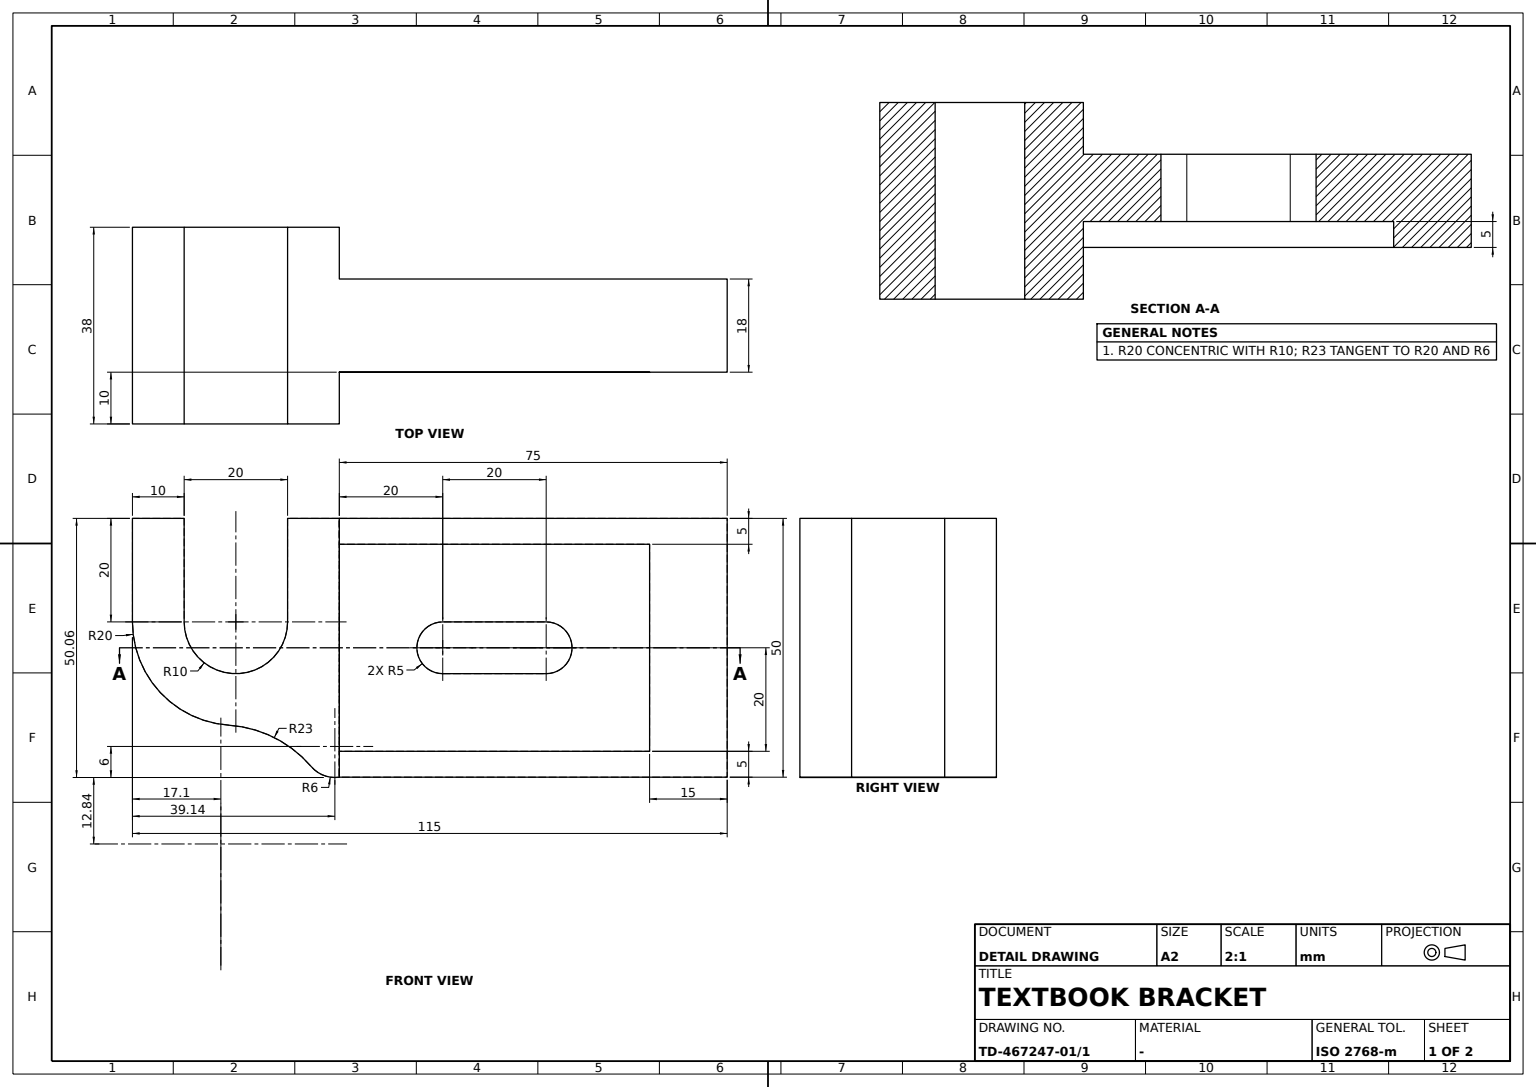
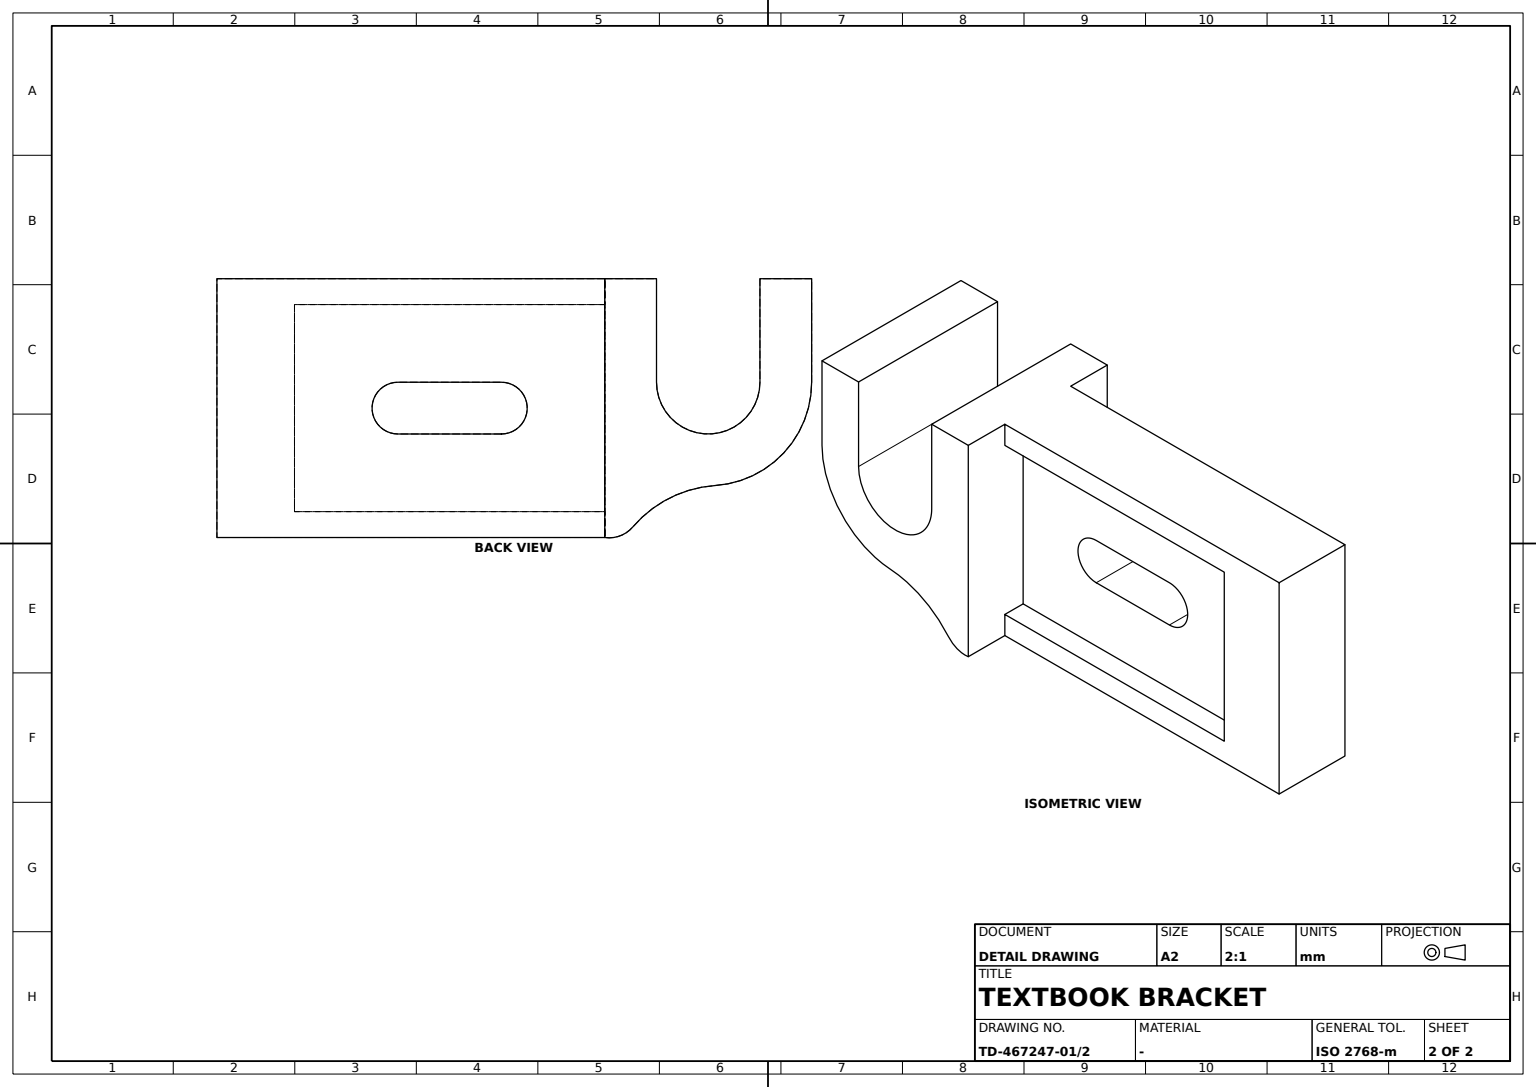
ISO-10303-21;
HEADER;
FILE_DESCRIPTION((''),'2;1');
FILE_NAME('','',(''),(''),'','','');
FILE_SCHEMA(('AUTOMOTIVE_DESIGN'));
ENDSEC;
DATA;
#1=APPLICATION_CONTEXT('');
#2=PRODUCT_CONTEXT('',#1,'mechanical');
#3=PRODUCT('','','',(#2));
#4=PRODUCT_DEFINITION_FORMATION('','',#3);
#5=PRODUCT_DEFINITION_CONTEXT('',#1,'design');
#6=PRODUCT_DEFINITION('','',#4,#5);
#7=PRODUCT_DEFINITION_SHAPE('','',#6);
#8=(LENGTH_UNIT()NAMED_UNIT(*)SI_UNIT(.MILLI.,.METRE.));
#9=(NAMED_UNIT(*)PLANE_ANGLE_UNIT()SI_UNIT($,.RADIAN.));
#10=(NAMED_UNIT(*)SI_UNIT($,.STERADIAN.)SOLID_ANGLE_UNIT());
#11=UNCERTAINTY_MEASURE_WITH_UNIT(LENGTH_MEASURE(0.005),#8,'distance_accuracy_value','');
#12=(GEOMETRIC_REPRESENTATION_CONTEXT(3)GLOBAL_UNCERTAINTY_ASSIGNED_CONTEXT((#11))GLOBAL_UNIT_ASSIGNED_CONTEXT((#8,#9,#10))REPRESENTATION_CONTEXT('',''));
#13=CARTESIAN_POINT('',(19.,-5.417023,-22.959402));
#14=VERTEX_POINT('',#13);
#15=CARTESIAN_POINT('',(19.,0.,-25.));
#16=VERTEX_POINT('',#15);
#17=CARTESIAN_POINT('',(19.,-0.85576,-19.061341));
#18=DIRECTION('',(1.,0.,0.));
#19=DIRECTION('',(0.,0.,-1.));
#20=AXIS2_PLACEMENT_3D('',#17,#18,#19);
#21=CIRCLE('',#20,6.);
#22=EDGE_CURVE('',#14,#16,#21,.T.);
#23=ORIENTED_EDGE('',*,*,#22,.F.);
#24=CARTESIAN_POINT('',(-19.,-5.417023,-22.959402));
#25=VERTEX_POINT('',#24);
#26=CARTESIAN_POINT('',(0.,-5.417023,-22.959402));
#27=VECTOR('',#18,1000.);
#28=LINE('',#26,#27);
#29=EDGE_CURVE('',#25,#14,#28,.T.);
#30=ORIENTED_EDGE('',*,*,#29,.F.);
#31=CARTESIAN_POINT('',(-19.,0.,-25.));
#32=VERTEX_POINT('',#31);
#33=CARTESIAN_POINT('',(-19.,-0.85576,-19.061341));
#34=AXIS2_PLACEMENT_3D('',#33,#18,#19);
#35=CIRCLE('',#34,6.);
#36=EDGE_CURVE('',#25,#32,#35,.T.);
#37=ORIENTED_EDGE('',*,*,#36,.T.);
#38=CARTESIAN_POINT('',(-9.,0.,-25.));
#39=VERTEX_POINT('',#38);
#40=LINE('',#31,#27);
#41=EDGE_CURVE('',#32,#39,#40,.T.);
#42=ORIENTED_EDGE('',*,*,#41,.T.);
#43=CARTESIAN_POINT('',(9.,0.,-25.));
#44=VERTEX_POINT('',#43);
#45=LINE('',#38,#27);
#46=EDGE_CURVE('',#39,#44,#45,.T.);
#47=ORIENTED_EDGE('',*,*,#46,.T.);
#48=LINE('',#43,#27);
#49=EDGE_CURVE('',#44,#16,#48,.T.);
#50=ORIENTED_EDGE('',*,*,#49,.T.);
#51=EDGE_LOOP('',(#23,#30,#37,#42,#47,#50));
#52=FACE_BOUND('',#51,.T.);
#53=CARTESIAN_POINT('',(0.,-0.85576,-19.061341));
#54=DIRECTION('',(0.,1.,0.));
#55=AXIS2_PLACEMENT_3D('',#53,#18,#54);
#56=CYLINDRICAL_SURFACE('',#55,6.);
#57=ADVANCED_FACE('',(#52),#56,.T.);
#58=CARTESIAN_POINT('',(-19.,-21.349703,-14.954406));
#59=VERTEX_POINT('',#58);
#60=CARTESIAN_POINT('',(19.,-21.349703,-14.954406));
#61=VERTEX_POINT('',#60);
#62=CARTESIAN_POINT('',(0.,-21.349703,-14.954406));
#63=LINE('',#62,#27);
#64=EDGE_CURVE('',#59,#61,#63,.T.);
#65=ORIENTED_EDGE('',*,*,#64,.T.);
#66=CARTESIAN_POINT('',(19.,-40.,5.));
#67=VERTEX_POINT('',#66);
#68=CARTESIAN_POINT('',(19.,-20.,5.));
#69=AXIS2_PLACEMENT_3D('',#68,#18,#19);
#70=CIRCLE('',#69,20.);
#71=EDGE_CURVE('',#67,#61,#70,.T.);
#72=ORIENTED_EDGE('',*,*,#71,.F.);
#73=CARTESIAN_POINT('',(-19.,-40.,5.));
#74=VERTEX_POINT('',#73);
#75=CARTESIAN_POINT('',(0.,-40.,5.));
#76=LINE('',#75,#27);
#77=EDGE_CURVE('',#74,#67,#76,.T.);
#78=ORIENTED_EDGE('',*,*,#77,.F.);
#79=CARTESIAN_POINT('',(-19.,-20.,5.));
#80=AXIS2_PLACEMENT_3D('',#79,#18,#19);
#81=CIRCLE('',#80,20.);
#82=EDGE_CURVE('',#74,#59,#81,.T.);
#83=ORIENTED_EDGE('',*,*,#82,.T.);
#84=EDGE_LOOP('',(#65,#72,#78,#83));
#85=FACE_BOUND('',#84,.T.);
#86=CARTESIAN_POINT('',(0.,-20.,5.));
#87=AXIS2_PLACEMENT_3D('',#86,#18,#54);
#88=CYLINDRICAL_SURFACE('',#87,20.);
#89=ADVANCED_FACE('',(#85),#88,.T.);
#90=CARTESIAN_POINT('',(4.,0.,20.));
#91=VERTEX_POINT('',#90);
#92=CARTESIAN_POINT('',(4.,60.,20.));
#93=VERTEX_POINT('',#92);
#94=VECTOR('',#54,1000.);
#95=LINE('',#90,#94);
#96=EDGE_CURVE('',#91,#93,#95,.T.);
#97=ORIENTED_EDGE('',*,*,#96,.T.);
#98=CARTESIAN_POINT('',(9.,60.,20.));
#99=VERTEX_POINT('',#98);
#100=DIRECTION('',(-1.,0.,0.));
#101=VECTOR('',#100,1000.);
#102=LINE('',#98,#101);
#103=EDGE_CURVE('',#99,#93,#102,.T.);
#104=ORIENTED_EDGE('',*,*,#103,.F.);
#105=CARTESIAN_POINT('',(9.,0.,20.));
#106=VERTEX_POINT('',#105);
#107=LINE('',#105,#94);
#108=EDGE_CURVE('',#106,#99,#107,.T.);
#109=ORIENTED_EDGE('',*,*,#108,.F.);
#110=LINE('',#105,#27);
#111=EDGE_CURVE('',#91,#106,#110,.T.);
#112=ORIENTED_EDGE('',*,*,#111,.F.);
#113=EDGE_LOOP('',(#97,#104,#109,#112));
#114=FACE_BOUND('',#113,.T.);
#115=DIRECTION('',(0.,0.,1.));
#116=AXIS2_PLACEMENT_3D('',#105,#115,#54);
#117=PLANE('',#116);
#118=ADVANCED_FACE('',(#114),#117,.F.);
#119=CARTESIAN_POINT('',(-19.,-10.,5.));
#120=VERTEX_POINT('',#119);
#121=CARTESIAN_POINT('',(-19.,-10.,25.));
#122=VERTEX_POINT('',#121);
#123=CARTESIAN_POINT('',(-19.,-10.,0.));
#124=VECTOR('',#115,1000.);
#125=LINE('',#123,#124);
#126=EDGE_CURVE('',#120,#122,#125,.T.);
#127=ORIENTED_EDGE('',*,*,#126,.F.);
#128=CARTESIAN_POINT('',(19.,-10.,5.));
#129=VERTEX_POINT('',#128);
#130=CARTESIAN_POINT('',(0.,-10.,5.));
#131=LINE('',#130,#27);
#132=EDGE_CURVE('',#120,#129,#131,.T.);
#133=ORIENTED_EDGE('',*,*,#132,.T.);
#134=CARTESIAN_POINT('',(19.,-10.,25.));
#135=VERTEX_POINT('',#134);
#136=CARTESIAN_POINT('',(19.,-10.,0.));
#137=LINE('',#136,#124);
#138=EDGE_CURVE('',#129,#135,#137,.T.);
#139=ORIENTED_EDGE('',*,*,#138,.T.);
#140=CARTESIAN_POINT('',(0.,-10.,25.));
#141=LINE('',#140,#27);
#142=EDGE_CURVE('',#122,#135,#141,.T.);
#143=ORIENTED_EDGE('',*,*,#142,.F.);
#144=EDGE_LOOP('',(#127,#133,#139,#143));
#145=FACE_BOUND('',#144,.T.);
#146=AXIS2_PLACEMENT_3D('',#130,#54,#115);
#147=PLANE('',#146);
#148=ADVANCED_FACE('',(#145),#147,.F.);
#149=CARTESIAN_POINT('',(9.,60.,-20.));
#150=VERTEX_POINT('',#149);
#151=VECTOR('',#19,1000.);
#152=LINE('',#98,#151);
#153=EDGE_CURVE('',#99,#150,#152,.T.);
#154=ORIENTED_EDGE('',*,*,#153,.F.);
#155=ORIENTED_EDGE('',*,*,#103,.T.);
#156=CARTESIAN_POINT('',(4.,60.,-20.));
#157=VERTEX_POINT('',#156);
#158=LINE('',#92,#151);
#159=EDGE_CURVE('',#93,#157,#158,.T.);
#160=ORIENTED_EDGE('',*,*,#159,.T.);
#161=LINE('',#149,#101);
#162=EDGE_CURVE('',#150,#157,#161,.T.);
#163=ORIENTED_EDGE('',*,*,#162,.F.);
#164=EDGE_LOOP('',(#154,#155,#160,#163));
#165=FACE_BOUND('',#164,.T.);
#166=AXIS2_PLACEMENT_3D('',#98,#54,#19);
#167=PLANE('',#166);
#168=ADVANCED_FACE('',(#165),#167,.F.);
#169=CARTESIAN_POINT('',(-9.,0.,25.));
#170=VERTEX_POINT('',#169);
#171=CARTESIAN_POINT('',(-9.,0.,0.));
#172=LINE('',#171,#151);
#173=EDGE_CURVE('',#170,#39,#172,.T.);
#174=ORIENTED_EDGE('',*,*,#173,.F.);
#175=CARTESIAN_POINT('',(-9.,75.,25.));
#176=VERTEX_POINT('',#175);
#177=LINE('',#169,#94);
#178=EDGE_CURVE('',#170,#176,#177,.T.);
#179=ORIENTED_EDGE('',*,*,#178,.T.);
#180=CARTESIAN_POINT('',(-9.,75.,-25.));
#181=VERTEX_POINT('',#180);
#182=CARTESIAN_POINT('',(-9.,75.,0.));
#183=LINE('',#182,#124);
#184=EDGE_CURVE('',#181,#176,#183,.T.);
#185=ORIENTED_EDGE('',*,*,#184,.F.);
#186=DIRECTION('',(0.,-1.,0.));
#187=VECTOR('',#186,1000.);
#188=LINE('',#38,#187);
#189=EDGE_CURVE('',#181,#39,#188,.T.);
#190=ORIENTED_EDGE('',*,*,#189,.T.);
#191=EDGE_LOOP('',(#174,#179,#185,#190));
#192=FACE_BOUND('',#191,.T.);
#193=CARTESIAN_POINT('',(-9.,20.,5.));
#194=VERTEX_POINT('',#193);
#195=CARTESIAN_POINT('',(-9.,40.,5.));
#196=VERTEX_POINT('',#195);
#197=LINE('',#193,#94);
#198=EDGE_CURVE('',#194,#196,#197,.T.);
#199=ORIENTED_EDGE('',*,*,#198,.F.);
#200=CARTESIAN_POINT('',(-9.,20.,-5.));
#201=VERTEX_POINT('',#200);
#202=CARTESIAN_POINT('',(-9.,20.,0.));
#203=AXIS2_PLACEMENT_3D('',#202,#18,#19);
#204=CIRCLE('',#203,5.);
#205=EDGE_CURVE('',#194,#201,#204,.T.);
#206=ORIENTED_EDGE('',*,*,#205,.T.);
#207=CARTESIAN_POINT('',(-9.,40.,-5.));
#208=VERTEX_POINT('',#207);
#209=LINE('',#200,#94);
#210=EDGE_CURVE('',#201,#208,#209,.T.);
#211=ORIENTED_EDGE('',*,*,#210,.T.);
#212=CARTESIAN_POINT('',(-9.,40.,0.));
#213=AXIS2_PLACEMENT_3D('',#212,#18,#19);
#214=CIRCLE('',#213,5.);
#215=EDGE_CURVE('',#208,#196,#214,.T.);
#216=ORIENTED_EDGE('',*,*,#215,.T.);
#217=EDGE_LOOP('',(#199,#206,#211,#216));
#218=FACE_BOUND('',#217,.T.);
#219=AXIS2_PLACEMENT_3D('',#171,#18,#54);
#220=PLANE('',#219);
#221=ADVANCED_FACE('',(#192,#218),#220,.F.);
#222=CARTESIAN_POINT('',(4.,40.,-5.));
#223=VERTEX_POINT('',#222);
#224=CARTESIAN_POINT('',(-3.16,40.,-5.));
#225=LINE('',#224,#27);
#226=EDGE_CURVE('',#223,#208,#225,.F.);
#227=ORIENTED_EDGE('',*,*,#226,.F.);
#228=CARTESIAN_POINT('',(4.,40.,5.));
#229=VERTEX_POINT('',#228);
#230=CARTESIAN_POINT('',(4.,40.,0.));
#231=AXIS2_PLACEMENT_3D('',#230,#18,#19);
#232=CIRCLE('',#231,5.);
#233=EDGE_CURVE('',#223,#229,#232,.T.);
#234=ORIENTED_EDGE('',*,*,#233,.T.);
#235=CARTESIAN_POINT('',(-3.16,40.,5.));
#236=LINE('',#235,#27);
#237=EDGE_CURVE('',#229,#196,#236,.F.);
#238=ORIENTED_EDGE('',*,*,#237,.T.);
#239=ORIENTED_EDGE('',*,*,#215,.F.);
#240=EDGE_LOOP('',(#227,#234,#238,#239));
#241=FACE_BOUND('',#240,.T.);
#242=CARTESIAN_POINT('',(-3.16,40.,0.));
#243=AXIS2_PLACEMENT_3D('',#242,#18,#54);
#244=CYLINDRICAL_SURFACE('',#243,5.);
#245=ADVANCED_FACE('',(#241),#244,.F.);
#246=CARTESIAN_POINT('',(9.,75.,25.));
#247=VERTEX_POINT('',#246);
#248=CARTESIAN_POINT('',(0.,75.,25.));
#249=LINE('',#248,#27);
#250=EDGE_CURVE('',#176,#247,#249,.T.);
#251=ORIENTED_EDGE('',*,*,#250,.T.);
#252=CARTESIAN_POINT('',(9.,75.,-25.));
#253=VERTEX_POINT('',#252);
#254=CARTESIAN_POINT('',(9.,75.,0.));
#255=LINE('',#254,#124);
#256=EDGE_CURVE('',#253,#247,#255,.T.);
#257=ORIENTED_EDGE('',*,*,#256,.F.);
#258=CARTESIAN_POINT('',(0.,75.,-25.));
#259=LINE('',#258,#27);
#260=EDGE_CURVE('',#181,#253,#259,.T.);
#261=ORIENTED_EDGE('',*,*,#260,.F.);
#262=ORIENTED_EDGE('',*,*,#184,.T.);
#263=EDGE_LOOP('',(#251,#257,#261,#262));
#264=FACE_BOUND('',#263,.T.);
#265=AXIS2_PLACEMENT_3D('',#258,#54,#115);
#266=PLANE('',#265);
#267=ADVANCED_FACE('',(#264),#266,.T.);
#268=CARTESIAN_POINT('',(-19.,-40.,25.));
#269=VERTEX_POINT('',#268);
#270=CARTESIAN_POINT('',(19.,-40.,25.));
#271=VERTEX_POINT('',#270);
#272=CARTESIAN_POINT('',(0.,-40.,25.));
#273=LINE('',#272,#27);
#274=EDGE_CURVE('',#269,#271,#273,.T.);
#275=ORIENTED_EDGE('',*,*,#274,.F.);
#276=CARTESIAN_POINT('',(-19.,-40.,0.));
#277=LINE('',#276,#124);
#278=EDGE_CURVE('',#74,#269,#277,.T.);
#279=ORIENTED_EDGE('',*,*,#278,.F.);
#280=ORIENTED_EDGE('',*,*,#77,.T.);
#281=CARTESIAN_POINT('',(19.,-40.,0.));
#282=LINE('',#281,#124);
#283=EDGE_CURVE('',#67,#271,#282,.T.);
#284=ORIENTED_EDGE('',*,*,#283,.T.);
#285=EDGE_LOOP('',(#275,#279,#280,#284));
#286=FACE_BOUND('',#285,.T.);
#287=AXIS2_PLACEMENT_3D('',#75,#54,#115);
#288=PLANE('',#287);
#289=ADVANCED_FACE('',(#286),#288,.F.);
#290=ORIENTED_EDGE('',*,*,#198,.T.);
#291=ORIENTED_EDGE('',*,*,#237,.F.);
#292=CARTESIAN_POINT('',(4.,20.,5.));
#293=VERTEX_POINT('',#292);
#294=LINE('',#292,#94);
#295=EDGE_CURVE('',#293,#229,#294,.T.);
#296=ORIENTED_EDGE('',*,*,#295,.F.);
#297=CARTESIAN_POINT('',(-3.16,20.,5.));
#298=LINE('',#297,#27);
#299=EDGE_CURVE('',#293,#194,#298,.F.);
#300=ORIENTED_EDGE('',*,*,#299,.T.);
#301=EDGE_LOOP('',(#290,#291,#296,#300));
#302=FACE_BOUND('',#301,.T.);
#303=AXIS2_PLACEMENT_3D('',#292,#115,#54);
#304=PLANE('',#303);
#305=ADVANCED_FACE('',(#302),#304,.F.);
#306=CARTESIAN_POINT('',(-19.,-30.,5.));
#307=VERTEX_POINT('',#306);
#308=CIRCLE('',#80,10.);
#309=EDGE_CURVE('',#307,#120,#308,.T.);
#310=ORIENTED_EDGE('',*,*,#309,.F.);
#311=CARTESIAN_POINT('',(19.,-30.,5.));
#312=VERTEX_POINT('',#311);
#313=CARTESIAN_POINT('',(0.,-30.,5.));
#314=LINE('',#313,#27);
#315=EDGE_CURVE('',#307,#312,#314,.T.);
#316=ORIENTED_EDGE('',*,*,#315,.T.);
#317=CIRCLE('',#69,10.);
#318=EDGE_CURVE('',#312,#129,#317,.T.);
#319=ORIENTED_EDGE('',*,*,#318,.T.);
#320=ORIENTED_EDGE('',*,*,#132,.F.);
#321=EDGE_LOOP('',(#310,#316,#319,#320));
#322=FACE_BOUND('',#321,.T.);
#323=CYLINDRICAL_SURFACE('',#87,10.);
#324=ADVANCED_FACE('',(#322),#323,.F.);
#325=CARTESIAN_POINT('',(4.,20.,-5.));
#326=VERTEX_POINT('',#325);
#327=CARTESIAN_POINT('',(4.,20.,0.));
#328=AXIS2_PLACEMENT_3D('',#327,#18,#19);
#329=CIRCLE('',#328,5.);
#330=EDGE_CURVE('',#293,#326,#329,.T.);
#331=ORIENTED_EDGE('',*,*,#330,.T.);
#332=CARTESIAN_POINT('',(-3.16,20.,-5.));
#333=LINE('',#332,#27);
#334=EDGE_CURVE('',#326,#201,#333,.F.);
#335=ORIENTED_EDGE('',*,*,#334,.T.);
#336=ORIENTED_EDGE('',*,*,#205,.F.);
#337=ORIENTED_EDGE('',*,*,#299,.F.);
#338=EDGE_LOOP('',(#331,#335,#336,#337));
#339=FACE_BOUND('',#338,.T.);
#340=CARTESIAN_POINT('',(-3.16,20.,0.));
#341=AXIS2_PLACEMENT_3D('',#340,#18,#54);
#342=CYLINDRICAL_SURFACE('',#341,5.);
#343=ADVANCED_FACE('',(#339),#342,.F.);
#344=ORIENTED_EDGE('',*,*,#64,.F.);
#345=CARTESIAN_POINT('',(-19.,-22.901862,-37.901972));
#346=AXIS2_PLACEMENT_3D('',#345,#18,#19);
#347=CIRCLE('',#346,23.);
#348=EDGE_CURVE('',#25,#59,#347,.T.);
#349=ORIENTED_EDGE('',*,*,#348,.F.);
#350=ORIENTED_EDGE('',*,*,#29,.T.);
#351=CARTESIAN_POINT('',(19.,-22.901862,-37.901972));
#352=AXIS2_PLACEMENT_3D('',#351,#18,#19);
#353=CIRCLE('',#352,23.);
#354=EDGE_CURVE('',#14,#61,#353,.T.);
#355=ORIENTED_EDGE('',*,*,#354,.T.);
#356=EDGE_LOOP('',(#344,#349,#350,#355));
#357=FACE_BOUND('',#356,.T.);
#358=CARTESIAN_POINT('',(0.,-22.901862,-37.901972));
#359=AXIS2_PLACEMENT_3D('',#358,#18,#54);
#360=CYLINDRICAL_SURFACE('',#359,23.);
#361=ADVANCED_FACE('',(#357),#360,.F.);
#362=CARTESIAN_POINT('',(9.,0.,25.));
#363=VERTEX_POINT('',#362);
#364=CARTESIAN_POINT('',(19.,0.,25.));
#365=VERTEX_POINT('',#364);
#366=CARTESIAN_POINT('',(0.,0.,25.));
#367=LINE('',#366,#27);
#368=EDGE_CURVE('',#363,#365,#367,.T.);
#369=ORIENTED_EDGE('',*,*,#368,.F.);
#370=LINE('',#362,#94);
#371=EDGE_CURVE('',#363,#247,#370,.T.);
#372=ORIENTED_EDGE('',*,*,#371,.T.);
#373=ORIENTED_EDGE('',*,*,#250,.F.);
#374=ORIENTED_EDGE('',*,*,#178,.F.);
#375=CARTESIAN_POINT('',(-19.,0.,25.));
#376=VERTEX_POINT('',#375);
#377=EDGE_CURVE('',#376,#170,#367,.T.);
#378=ORIENTED_EDGE('',*,*,#377,.F.);
#379=LINE('',#375,#94);
#380=EDGE_CURVE('',#122,#376,#379,.T.);
#381=ORIENTED_EDGE('',*,*,#380,.F.);
#382=ORIENTED_EDGE('',*,*,#142,.T.);
#383=LINE('',#364,#94);
#384=EDGE_CURVE('',#135,#365,#383,.T.);
#385=ORIENTED_EDGE('',*,*,#384,.T.);
#386=EDGE_LOOP('',(#369,#372,#373,#374,#378,#381,#382,#385));
#387=FACE_BOUND('',#386,.T.);
#388=AXIS2_PLACEMENT_3D('',#366,#19,#54);
#389=PLANE('',#388);
#390=ADVANCED_FACE('',(#387),#389,.F.);
#391=CARTESIAN_POINT('',(19.,-30.,25.));
#392=VERTEX_POINT('',#391);
#393=CARTESIAN_POINT('',(19.,-30.,0.));
#394=LINE('',#393,#124);
#395=EDGE_CURVE('',#312,#392,#394,.T.);
#396=ORIENTED_EDGE('',*,*,#395,.F.);
#397=ORIENTED_EDGE('',*,*,#315,.F.);
#398=CARTESIAN_POINT('',(-19.,-30.,25.));
#399=VERTEX_POINT('',#398);
#400=CARTESIAN_POINT('',(-19.,-30.,0.));
#401=LINE('',#400,#124);
#402=EDGE_CURVE('',#307,#399,#401,.T.);
#403=ORIENTED_EDGE('',*,*,#402,.T.);
#404=CARTESIAN_POINT('',(0.,-30.,25.));
#405=LINE('',#404,#27);
#406=EDGE_CURVE('',#399,#392,#405,.T.);
#407=ORIENTED_EDGE('',*,*,#406,.T.);
#408=EDGE_LOOP('',(#396,#397,#403,#407));
#409=FACE_BOUND('',#408,.T.);
#410=AXIS2_PLACEMENT_3D('',#313,#54,#115);
#411=PLANE('',#410);
#412=ADVANCED_FACE('',(#409),#411,.T.);
#413=ORIENTED_EDGE('',*,*,#334,.F.);
#414=LINE('',#325,#94);
#415=EDGE_CURVE('',#326,#223,#414,.T.);
#416=ORIENTED_EDGE('',*,*,#415,.T.);
#417=ORIENTED_EDGE('',*,*,#226,.T.);
#418=ORIENTED_EDGE('',*,*,#210,.F.);
#419=EDGE_LOOP('',(#413,#416,#417,#418));
#420=FACE_BOUND('',#419,.T.);
#421=AXIS2_PLACEMENT_3D('',#325,#115,#54);
#422=PLANE('',#421);
#423=ADVANCED_FACE('',(#420),#422,.T.);
#424=ORIENTED_EDGE('',*,*,#415,.F.);
#425=ORIENTED_EDGE('',*,*,#330,.F.);
#426=ORIENTED_EDGE('',*,*,#295,.T.);
#427=ORIENTED_EDGE('',*,*,#233,.F.);
#428=EDGE_LOOP('',(#424,#425,#426,#427));
#429=FACE_BOUND('',#428,.T.);
#430=ORIENTED_EDGE('',*,*,#96,.F.);
#431=CARTESIAN_POINT('',(4.,0.,-20.));
#432=VERTEX_POINT('',#431);
#433=CARTESIAN_POINT('',(4.,0.,0.));
#434=LINE('',#433,#151);
#435=EDGE_CURVE('',#91,#432,#434,.T.);
#436=ORIENTED_EDGE('',*,*,#435,.T.);
#437=LINE('',#156,#187);
#438=EDGE_CURVE('',#157,#432,#437,.T.);
#439=ORIENTED_EDGE('',*,*,#438,.F.);
#440=ORIENTED_EDGE('',*,*,#159,.F.);
#441=EDGE_LOOP('',(#430,#436,#439,#440));
#442=FACE_BOUND('',#441,.T.);
#443=AXIS2_PLACEMENT_3D('',#433,#18,#54);
#444=PLANE('',#443);
#445=ADVANCED_FACE('',(#429,#442),#444,.T.);
#446=ORIENTED_EDGE('',*,*,#126,.T.);
#447=ORIENTED_EDGE('',*,*,#380,.T.);
#448=CARTESIAN_POINT('',(-19.,0.,0.));
#449=LINE('',#448,#151);
#450=EDGE_CURVE('',#376,#32,#449,.T.);
#451=ORIENTED_EDGE('',*,*,#450,.T.);
#452=ORIENTED_EDGE('',*,*,#36,.F.);
#453=ORIENTED_EDGE('',*,*,#348,.T.);
#454=ORIENTED_EDGE('',*,*,#82,.F.);
#455=ORIENTED_EDGE('',*,*,#278,.T.);
#456=EDGE_CURVE('',#269,#399,#379,.T.);
#457=ORIENTED_EDGE('',*,*,#456,.T.);
#458=ORIENTED_EDGE('',*,*,#402,.F.);
#459=ORIENTED_EDGE('',*,*,#309,.T.);
#460=EDGE_LOOP('',(#446,#447,#451,#452,#453,#454,#455,#457,#458,#459));
#461=FACE_BOUND('',#460,.T.);
#462=AXIS2_PLACEMENT_3D('',#448,#18,#54);
#463=PLANE('',#462);
#464=ADVANCED_FACE('',(#461),#463,.F.);
#465=CARTESIAN_POINT('',(9.,0.,-20.));
#466=VERTEX_POINT('',#465);
#467=LINE('',#149,#187);
#468=EDGE_CURVE('',#150,#466,#467,.T.);
#469=ORIENTED_EDGE('',*,*,#468,.F.);
#470=ORIENTED_EDGE('',*,*,#162,.T.);
#471=ORIENTED_EDGE('',*,*,#438,.T.);
#472=CARTESIAN_POINT('',(0.,0.,-20.));
#473=LINE('',#472,#27);
#474=EDGE_CURVE('',#432,#466,#473,.T.);
#475=ORIENTED_EDGE('',*,*,#474,.T.);
#476=EDGE_LOOP('',(#469,#470,#471,#475));
#477=FACE_BOUND('',#476,.T.);
#478=AXIS2_PLACEMENT_3D('',#149,#19,#186);
#479=PLANE('',#478);
#480=ADVANCED_FACE('',(#477),#479,.F.);
#481=ORIENTED_EDGE('',*,*,#173,.T.);
#482=ORIENTED_EDGE('',*,*,#41,.F.);
#483=ORIENTED_EDGE('',*,*,#450,.F.);
#484=ORIENTED_EDGE('',*,*,#377,.T.);
#485=EDGE_LOOP('',(#481,#482,#483,#484));
#486=FACE_BOUND('',#485,.T.);
#487=AXIS2_PLACEMENT_3D('',#366,#186,#19);
#488=PLANE('',#487);
#489=ADVANCED_FACE('',(#486),#488,.F.);
#490=ORIENTED_EDGE('',*,*,#189,.F.);
#491=ORIENTED_EDGE('',*,*,#260,.T.);
#492=LINE('',#43,#187);
#493=EDGE_CURVE('',#253,#44,#492,.T.);
#494=ORIENTED_EDGE('',*,*,#493,.T.);
#495=ORIENTED_EDGE('',*,*,#46,.F.);
#496=EDGE_LOOP('',(#490,#491,#494,#495));
#497=FACE_BOUND('',#496,.T.);
#498=AXIS2_PLACEMENT_3D('',#258,#115,#186);
#499=PLANE('',#498);
#500=ADVANCED_FACE('',(#497),#499,.F.);
#501=ORIENTED_EDGE('',*,*,#49,.F.);
#502=CARTESIAN_POINT('',(9.,0.,0.));
#503=LINE('',#502,#151);
#504=EDGE_CURVE('',#466,#44,#503,.T.);
#505=ORIENTED_EDGE('',*,*,#504,.F.);
#506=ORIENTED_EDGE('',*,*,#474,.F.);
#507=ORIENTED_EDGE('',*,*,#435,.F.);
#508=ORIENTED_EDGE('',*,*,#111,.T.);
#509=EDGE_CURVE('',#363,#106,#503,.T.);
#510=ORIENTED_EDGE('',*,*,#509,.F.);
#511=ORIENTED_EDGE('',*,*,#368,.T.);
#512=CARTESIAN_POINT('',(19.,0.,0.));
#513=LINE('',#512,#151);
#514=EDGE_CURVE('',#365,#16,#513,.T.);
#515=ORIENTED_EDGE('',*,*,#514,.T.);
#516=EDGE_LOOP('',(#501,#505,#506,#507,#508,#510,#511,#515));
#517=FACE_BOUND('',#516,.T.);
#518=ADVANCED_FACE('',(#517),#488,.F.);
#519=ORIENTED_EDGE('',*,*,#456,.F.);
#520=ORIENTED_EDGE('',*,*,#274,.T.);
#521=EDGE_CURVE('',#271,#392,#383,.T.);
#522=ORIENTED_EDGE('',*,*,#521,.T.);
#523=ORIENTED_EDGE('',*,*,#406,.F.);
#524=EDGE_LOOP('',(#519,#520,#522,#523));
#525=FACE_BOUND('',#524,.T.);
#526=ADVANCED_FACE('',(#525),#389,.F.);
#527=ORIENTED_EDGE('',*,*,#493,.F.);
#528=ORIENTED_EDGE('',*,*,#256,.T.);
#529=ORIENTED_EDGE('',*,*,#371,.F.);
#530=ORIENTED_EDGE('',*,*,#509,.T.);
#531=ORIENTED_EDGE('',*,*,#108,.T.);
#532=ORIENTED_EDGE('',*,*,#153,.T.);
#533=ORIENTED_EDGE('',*,*,#468,.T.);
#534=ORIENTED_EDGE('',*,*,#504,.T.);
#535=EDGE_LOOP('',(#527,#528,#529,#530,#531,#532,#533,#534));
#536=FACE_BOUND('',#535,.T.);
#537=AXIS2_PLACEMENT_3D('',#502,#18,#54);
#538=PLANE('',#537);
#539=ADVANCED_FACE('',(#536),#538,.T.);
#540=ORIENTED_EDGE('',*,*,#22,.T.);
#541=ORIENTED_EDGE('',*,*,#514,.F.);
#542=ORIENTED_EDGE('',*,*,#384,.F.);
#543=ORIENTED_EDGE('',*,*,#138,.F.);
#544=ORIENTED_EDGE('',*,*,#318,.F.);
#545=ORIENTED_EDGE('',*,*,#395,.T.);
#546=ORIENTED_EDGE('',*,*,#521,.F.);
#547=ORIENTED_EDGE('',*,*,#283,.F.);
#548=ORIENTED_EDGE('',*,*,#71,.T.);
#549=ORIENTED_EDGE('',*,*,#354,.F.);
#550=EDGE_LOOP('',(#540,#541,#542,#543,#544,#545,#546,#547,#548,#549));
#551=FACE_BOUND('',#550,.T.);
#552=AXIS2_PLACEMENT_3D('',#512,#18,#54);
#553=PLANE('',#552);
#554=ADVANCED_FACE('',(#551),#553,.T.);
#555=CLOSED_SHELL('',(#57,#89,#118,#148,#168,#221,#245,#267,#289,#305,#324,#343,#361,#390,#412,#423,#445,#464,#480,#489,#500,#518,#526,#539,#554));
#556=MANIFOLD_SOLID_BREP('',#555);
#557=ADVANCED_BREP_SHAPE_REPRESENTATION('',(#556),#12);
#558=SHAPE_DEFINITION_REPRESENTATION(#7,#557);
ENDSEC;
END-ISO-10303-21;
